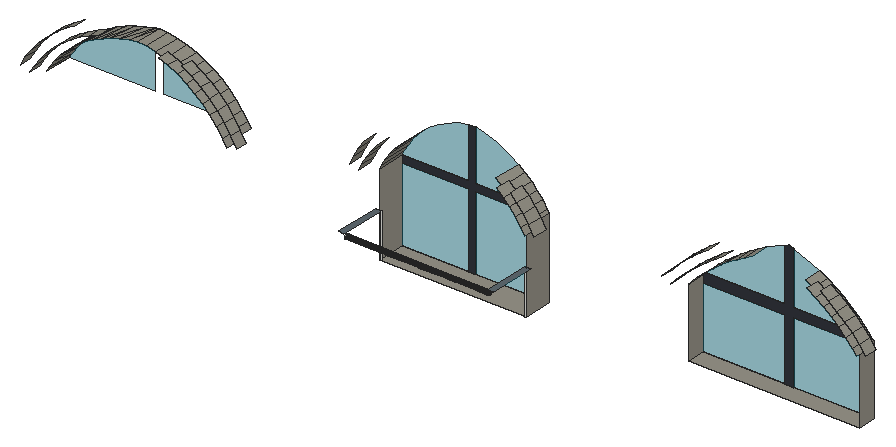
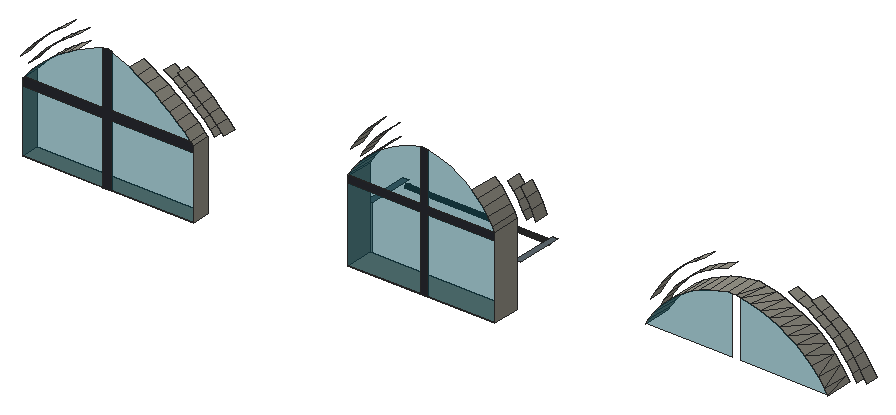
# SketchUp Ruby script. Lengths in inches.
U = 1.inch
M = Sketchup.active_model
def pt(a) = Geom::Point3d.new(a.map { |v| v * U })
def face(e, loops, mat)
  f = e.add_face(loops[0].map { |a| pt(a) })
  loops[1..].each { |l| e.add_face(l.map { |a| pt(a) }).erase! }
  f.material = f.back_material = mat if mat
  f
end
# faces: each face lists its corners as indices into pts; further lists are holes
def faces(e, pts, list, mat = nil) = list.each { |f| face(e, (f[0].is_a?(Array) ? f : [f]).map { |l| l.map { |i| pts[i] } }, mat) }
# xy, xz, yz: faces in a plane at the given z, y or x. An outline is a flat list of corners, or four numbers for a rectangle; further outlines are holes
def ring(l) = l.size == 4 ? [[l[0], l[1]], [l[2], l[1]], [l[2], l[3]], [l[0], l[3]]] : l.each_slice(2).to_a
def flat(e, list, mat, &to3) = list.each { |f| face(e, (f[0].is_a?(Array) ? f : [f]).map { |l| ring(l).map { |u, v| to3.(u, v) } }, mat) }
def xy(e, z, list, mat = nil) = flat(e, list, mat) { |x, y| [x, y, z] }
def xz(e, y, list, mat = nil) = flat(e, list, mat) { |x, z| [x, y, z] }
def yz(e, x, list, mat = nil) = flat(e, list, mat) { |y, z| [x, y, z] }
def lines(e, pts, list) = list.each { |a, b| e.add_line(pt(pts[a]), pt(pts[b])) }
# prism: a flat outline (further loops are holes) pulled along v
def prism(e, loops, v, mat = nil)
  f = face(e, loops, mat); d = Geom::Vector3d.new(v.map { |x| x * U })
  f.pushpull(f.normal.samedirection?(d) ? d.length : -d.length)
end
def box(e, o, s, mat = nil) = prism(e, [[o, [o[0] + s[0], o[1], o[2]], [o[0] + s[0], o[1] + s[1], o[2]], [o[0], o[1] + s[1], o[2]]]], [0, 0, s[2]], mat)
def at(x, y, z, deg = 0) = Geom::Transformation.translation(pt([x, y, z])) * Geom::Transformation.rotation(ORIGIN, Z_AXIS, deg.degrees)
def axes(o, x, y, z) = Geom::Transformation.new([*x, 0, *y, 0, *z, 0, *pt(o).to_a, 1])
def part(name) = M.definitions.add(name)
# library, detail: a bought-in or finely detailed component or shape, given as its bounding box
def library(name, o, s) = part(name).tap { |d| box(d.entities, o, s) }
def detail(e, o, s) = box(e.add_group.entities, o, s)
def put(e, d, t, mat = nil) = e.add_instance(d, t).tap { |i| i.material = mat if mat }
def group(e, t, mat = nil) = e.add_group.tap { |g| g.transformation = t; g.material = mat if mat }.entities
root = M.entities
M.materials.add("[Color M07]").color = [58, 58, 58]
M.materials.add("[Formica Graystone]").color = [149, 146, 135]
M.materials.add("[Formica Laminate Dark]").color = [50, 53, 60]
M.materials.add("[Formica Speckled Grey]").color = [94, 105, 111]
M.materials.add("[Translucent Glass Tinted]").color = [4, 106, 127]
M.materials["[Translucent Glass Tinted]"].alpha = 0.48
xy(root,336.52,[[366.31,158.3,451.49,167.05]],"[Formica Graystone]")
xy(root,337.93,[[223.375,144.04,296.73,158.1]],"[Formica Graystone]")
xy(root,357.6,[[226.04,121.51,226.22,121.51,226.4,121.55,226.55,121.64,226.68,121.76,226.77,121.92,226.82,122.09,226.82,122.27,226.78,122.45,226.6875,122.6,226.5625,122.73,226.41,122.82,226.23,122.87,226.06,122.87,225.88,122.83,225.73,122.74,225.6,122.61,225.51,122.46,225.46,122.28,225.46,122.11,225.5,121.93,225.59,121.78,225.71,121.65,225.87,121.56]])
xy(root,357.67,[[291.54,121.51,291.72,121.51,291.9,121.55,292.05,121.64,292.18,121.76,292.27,121.92,292.32,122.09,292.32,122.27,292.28,122.45,292.1875,122.6,292.0625,122.73,291.91,122.82,291.73,122.87,291.56,122.87,291.38,122.83,291.23,122.74,291.1,122.61,291.01,122.46,290.96,122.28,290.96,122.11,291,121.93,291.09,121.78,291.21,121.65,291.37,121.56]])
xy(root,357.79,[[248.54,121.51,248.72,121.51,248.9,121.55,249.05,121.64,249.18,121.76,249.27,121.92,249.32,122.09,249.32,122.27,249.28,122.45,249.1875,122.6,249.0625,122.73,248.91,122.82,248.73,122.87,248.56,122.87,248.38,122.83,248.23,122.74,248.1,122.61,248.01,122.46,247.96,122.28,247.96,122.11,248,121.93,248.09,121.78,248.21,121.65,248.37,121.56]])
xy(root,357.82,[[288.85,121.51,289.03,121.51,289.21,121.55,289.36,121.64,289.49,121.76,289.58,121.92,289.63,122.09,289.63,122.27,289.59,122.45,289.5,122.6,289.375,122.73,289.22,122.82,289.05,122.87,288.87,122.87,288.69,122.83,288.54,122.74,288.41,122.61,288.32,122.46,288.27,122.28,288.27,122.11,288.3125,121.93,288.4,121.78,288.53,121.65,288.68,121.56]])
xy(root,358.04,[[294.1,121.51,294.28,121.51,294.46,121.55,294.61,121.64,294.74,121.76,294.83,121.92,294.88,122.09,294.88,122.27,294.84,122.45,294.75,122.6,294.625,122.73,294.47,122.82,294.3,122.87,294.12,122.87,293.94,122.83,293.79,122.74,293.66,122.61,293.57,122.46,293.52,122.28,293.52,122.11,293.5625,121.93,293.65,121.78,293.78,121.65,293.93,121.56]])
xy(root,358.07,[[228.85,121.51,229.03,121.51,229.21,121.55,229.36,121.64,229.49,121.76,229.58,121.92,229.63,122.09,229.63,122.27,229.59,122.45,229.5,122.6,229.375,122.73,229.22,122.82,229.05,122.87,228.87,122.87,228.69,122.83,228.54,122.74,228.41,122.61,228.32,122.46,228.27,122.28,228.27,122.11,228.3125,121.93,228.4,121.78,228.53,121.65,228.68,121.56],[242.92,121.51,243.1,121.51,243.27,121.55,243.43,121.64,243.55,121.76,243.65,121.92,243.69,122.09,243.7,122.27,243.65,122.45,243.5625,122.6,243.4375,122.73,243.28,122.82,243.11,122.87,242.93,122.87,242.76,122.83,242.6,122.74,242.47,122.61,242.38,122.46,242.33,122.28,242.33,122.11,242.375,121.93,242.46,121.78,242.59,121.65,242.74,121.56],[245.73,121.51,245.91,121.51,246.08,121.55,246.24,121.64,246.37,121.76,246.46,121.92,246.51,122.09,246.51,122.27,246.46,122.45,246.375,122.6,246.25,122.73,246.1,122.82,245.92,122.87,245.74,122.87,245.57,122.83,245.41,122.74,245.28,122.61,245.19,122.46,245.15,122.28,245.14,122.11,245.1875,121.93,245.28,121.78,245.4,121.65,245.56,121.56],[251.29,121.51,251.47,121.51,251.65,121.55,251.8,121.64,251.93,121.76,252.02,121.92,252.07,122.09,252.07,122.27,252.03,122.45,251.9375,122.6,251.8125,122.73,251.66,122.82,251.48,122.87,251.31,122.87,251.13,122.83,250.98,122.74,250.85,122.61,250.76,122.46,250.71,122.28,250.71,122.11,250.75,121.93,250.84,121.78,250.96,121.65,251.12,121.56],[267.79,121.51,267.97,121.51,268.15,121.55,268.3,121.64,268.43,121.76,268.52,121.92,268.57,122.09,268.57,122.27,268.53,122.45,268.4375,122.6,268.3125,122.73,268.16,122.82,267.98,122.87,267.81,122.87,267.63,122.83,267.48,122.74,267.35,122.61,267.26,122.46,267.21,122.28,267.21,122.11,267.25,121.93,267.34,121.78,267.46,121.65,267.62,121.56],
  [270.54,121.51,270.72,121.51,270.9,121.55,271.05,121.64,271.18,121.76,271.27,121.92,271.32,122.09,271.32,122.27,271.28,122.45,271.1875,122.6,271.0625,122.73,270.91,122.82,270.73,122.87,270.56,122.87,270.38,122.83,270.23,122.74,270.1,122.61,270.01,122.46,269.96,122.28,269.96,122.11,270,121.93,270.09,121.78,270.21,121.65,270.37,121.56],[273.48,121.51,273.66,121.51,273.83,121.55,273.99,121.64,274.12,121.76,274.21,121.92,274.26,122.09,274.26,122.27,274.21,122.45,274.125,122.6,274,122.73,273.85,122.82,273.67,122.87,273.49,122.87,273.32,122.83,273.16,122.74,273.03,122.61,272.94,122.46,272.9,122.28,272.89,122.11,272.9375,121.93,273.03,121.78,273.15,121.65,273.31,121.56],[285.92,121.51,286.1,121.51,286.27,121.55,286.43,121.64,286.55,121.76,286.65,121.92,286.69,122.09,286.7,122.27,286.65,122.45,286.5625,122.6,286.4375,122.73,286.28,122.82,286.11,122.87,285.93,122.87,285.76,122.83,285.6,122.74,285.47,122.61,285.38,122.46,285.33,122.28,285.33,122.11,285.375,121.93,285.46,121.78,285.59,121.65,285.74,121.56]])
xy(root,358.23,[[279.04,121.51,279.22,121.51,279.4,121.55,279.55,121.64,279.68,121.76,279.77,121.92,279.82,122.09,279.82,122.27,279.78,122.45,279.6875,122.6,279.5625,122.73,279.41,122.82,279.23,122.87,279.06,122.87,278.88,122.83,278.73,122.74,278.6,122.61,278.51,122.46,278.46,122.28,278.46,122.11,278.5,121.93,278.59,121.78,278.71,121.65,278.87,121.56]])
xy(root,358.31,[[231.67,121.51,231.85,121.51,232.02,121.55,232.18,121.64,232.3,121.76,232.4,121.92,232.44,122.09,232.45,122.27,232.4,122.45,232.3125,122.6,232.1875,122.73,232.03,122.82,231.86,122.87,231.68,122.87,231.51,122.83,231.35,122.74,231.22,122.61,231.13,122.46,231.08,122.28,231.08,122.11,231.125,121.93,231.21,121.78,231.34,121.65,231.49,121.56],[234.48,121.51,234.66,121.51,234.83,121.55,234.99,121.64,235.12,121.76,235.21,121.92,235.26,122.09,235.26,122.27,235.21,122.45,235.125,122.6,235,122.73,234.85,122.82,234.67,122.87,234.49,122.87,234.32,122.83,234.16,122.74,234.03,122.61,233.94,122.46,233.9,122.28,233.89,122.11,233.9375,121.93,234.03,121.78,234.15,121.65,234.31,121.56],[254.04,121.51,254.22,121.51,254.4,121.55,254.55,121.64,254.68,121.76,254.77,121.92,254.82,122.09,254.82,122.27,254.78,122.45,254.6875,122.6,254.5625,122.73,254.41,122.82,254.23,122.87,254.06,122.87,253.88,122.83,253.73,122.74,253.6,122.61,253.51,122.46,253.46,122.28,253.46,122.11,253.5,121.93,253.59,121.78,253.71,121.65,253.87,121.56],[256.79,121.51,256.97,121.51,257.15,121.55,257.3,121.64,257.43,121.76,257.52,121.92,257.57,122.09,257.57,122.27,257.53,122.45,257.4375,122.6,257.3125,122.73,257.16,122.82,256.98,122.87,256.81,122.87,256.63,122.83,256.48,122.74,256.35,122.61,256.26,122.46,256.21,122.28,256.21,122.11,256.25,121.93,256.34,121.78,256.46,121.65,256.62,121.56],[259.54,121.51,259.72,121.51,259.9,121.55,260.05,121.64,260.18,121.76,260.27,121.92,260.32,122.09,260.32,122.27,260.28,122.45,260.1875,122.6,260.0625,122.73,259.91,122.82,259.73,122.87,259.56,122.87,259.38,122.83,259.23,122.74,259.1,122.61,259.01,122.46,258.96,122.28,258.96,122.11,259,121.93,259.09,121.78,259.21,121.65,259.37,121.56],
  [262.29,121.51,262.47,121.51,262.65,121.55,262.8,121.64,262.93,121.76,263.02,121.92,263.07,122.09,263.07,122.27,263.03,122.45,262.9375,122.6,262.8125,122.73,262.66,122.82,262.48,122.87,262.31,122.87,262.13,122.83,261.98,122.74,261.85,122.61,261.76,122.46,261.71,122.28,261.71,122.11,261.75,121.93,261.84,121.78,261.96,121.65,262.12,121.56],[282.29,121.51,282.47,121.51,282.65,121.55,282.8,121.64,282.93,121.76,283.02,121.92,283.07,122.09,283.07,122.27,283.03,122.45,282.9375,122.6,282.8125,122.73,282.66,122.82,282.48,122.87,282.31,122.87,282.13,122.83,281.98,122.74,281.85,122.61,281.76,122.46,281.71,122.28,281.71,122.11,281.75,121.93,281.84,121.78,281.96,121.65,282.12,121.56]])
xy(root,358.53,[[237.29,121.51,237.47,121.51,237.65,121.55,237.8,121.64,237.93,121.76,238.02,121.92,238.07,122.09,238.07,122.27,238.03,122.45,237.9375,122.6,237.8125,122.73,237.66,122.82,237.48,122.87,237.31,122.87,237.13,122.83,236.98,122.74,236.85,122.61,236.76,122.46,236.71,122.28,236.71,122.11,236.75,121.93,236.84,121.78,236.96,121.65,237.12,121.56],[240.1,121.51,240.28,121.51,240.46,121.55,240.61,121.64,240.74,121.76,240.83,121.92,240.88,122.09,240.88,122.27,240.84,122.45,240.75,122.6,240.625,122.73,240.47,122.82,240.3,122.87,240.12,122.87,239.94,122.83,239.79,122.74,239.66,122.61,239.57,122.46,239.52,122.28,239.52,122.11,239.5625,121.93,239.65,121.78,239.78,121.65,239.93,121.56],[265.04,121.51,265.22,121.51,265.4,121.55,265.55,121.64,265.68,121.76,265.77,121.92,265.82,122.09,265.82,122.27,265.78,122.45,265.6875,122.6,265.5625,122.73,265.41,122.82,265.23,122.87,265.06,122.87,264.88,122.83,264.73,122.74,264.6,122.61,264.51,122.46,264.46,122.28,264.46,122.11,264.5,121.93,264.59,121.78,264.71,121.65,264.87,121.56],[276.29,121.51,276.47,121.51,276.65,121.55,276.8,121.64,276.93,121.76,277.02,121.92,277.07,122.09,277.07,122.27,277.03,122.45,276.9375,122.6,276.8125,122.73,276.66,122.82,276.48,122.87,276.31,122.87,276.13,122.83,275.98,122.74,275.85,122.61,275.76,122.46,275.71,122.28,275.71,122.11,275.75,121.93,275.84,121.78,275.96,121.65,276.12,121.56]])
xy(root,359.98,[[221.4,120.91,224.22,144.04],[295.92,120.91,298.73,144.04]],"[Formica Speckled Grey]")
xz(root,144.04,[[223.375,337.93,224.22,359.98],[295.92,337.93,296.73,359.98]])
xz(root,157.6,[[57.22,363.79,100.86,363.79,100.86,392.22,95.875,391.25,90.98,389.9,86.22,388.15,81.61,386.02,77.1875,383.53,72.98,380.69,69.01,377.52,65.32,374.05,61.91,370.28,58.82,366.26],[104.96,363.79,148.1,363.79,148.1,363.97,146.62,366.62,143.875,370.65,140.79,374.42,137.39,377.91,133.69,381.08,129.73,383.92,125.53,386.4,121.14,388.5,116.57,390.21,111.875,391.51,107.08,392.39,104.96,392.59]],"[Translucent Glass Tinted]")
xz(root,158.1,[[256.49,337.93,260.1,337.93,260.1,374.93,296.73,374.93,296.73,377.84,296.41,378.37,260.1,378.37,260.1,403.77,259.55,403.88,256.49,403.57,256.49,378.37,223.375,378.37,223.375,374.93,256.49,374.93]],"[Formica Laminate Dark]")
xz(root,158.1,[[223.375,337.93,256.49,374.93],[260.1,337.93,296.73,374.93],[223.375,378.37,256.49,378.37,256.49,403.57,252.47,402.78,248.55,401.61,244.76,400.07,241.125,398.18,237.6875,395.96,234.47,393.42,231.52,390.6,228.84,387.5,226.46,384.17,224.41,380.625],[260.1,378.37,296.41,378.37,295.73,379.52,293.33,382.9375,290.6875,386.17,287.8,389.1875,284.7,391.99,281.4,394.54,277.91,396.84,274.27,398.875,270.47,400.625,266.5625,402.09,262.55,403.25,260.1,403.77]],"[Translucent Glass Tinted]")
xz(root,167.05,[[407.09,336.52,411.36,336.52,411.36,367.77,451.49,367.77,451.49,371.35,450.74,372.28,411.36,372.28,411.36,398.78,409.2,399.41,407.09,398.63,407.09,372.28,367.48,372.28,366.31,371.02,366.31,367.77,407.09,367.77]],"[Formica Laminate Dark]")
xz(root,167.05,[[366.31,336.52,407.09,367.77],[411.36,336.52,451.49,367.77],[367.48,372.28,407.09,372.28,407.09,398.63,402.67,396.78,398.33,394.75,394.08,392.53,389.92,390.13,385.88,387.56,381.94,384.83,378.13,381.92,374.44,378.86,370.89,375.64],[411.36,372.28,450.74,372.28,450.21,372.9375,447.04,376.44,443.68,379.77,440.15,382.91,436.44,385.84,432.58,388.57,428.58,391.07,424.4375,393.36,420.18,395.41,415.8125,397.22,411.36,398.78]],"[Translucent Glass Tinted]")
yz(root,223.375,[[144.04,337.93,158.1,378.37]],"[Formica Graystone]")
yz(root,224.22,[[122.22,357.13,121.97,357.16,121.75,357.25,121.55,357.4,121.41,357.6,121.3125,357.82,121.28,358.07,121.3125,358.31,121.41,358.53,121.55,358.73,121.75,358.88,121.97,358.97,122.22,359,122.46,358.97,122.6875,358.88,122.88,358.73,123.03,358.53,123.125,358.31,123.16,358.07,123.125,357.82,123.03,357.6,122.88,357.4,122.6875,357.25,122.46,357.16]])
yz(root,296.73,[[144.04,337.93,158.1,377.84]],"[Formica Graystone]")
yz(root,366.31,[[158.3,336.52,167.05,371.02]],"[Formica Graystone]")
yz(root,451.49,[[158.3,336.52,167.05,371.35]],"[Formica Graystone]")
p = [[224.22,121.97,357.16],[224.22,122.22,357.13],[295.92,122.22,357.13],[295.92,121.97,357.16],[224.22,122.46,357.16],[295.92,122.46,357.16],
  [224.22,121.75,357.25],[295.92,121.75,357.25],[224.22,122.6875,357.25],[295.92,122.6875,357.25],[224.22,121.55,357.4],[295.92,121.55,357.4],
  [293.93,121.56,357.4],[291.37,121.56,357.4],[288.68,121.56,357.4],[285.74,121.56,357.4],[282.12,121.56,357.4],[278.87,121.56,357.4],
  [276.12,121.56,357.4],[273.31,121.56,357.4],[270.37,121.56,357.4],[267.62,121.56,357.4],[264.87,121.56,357.4],[262.12,121.56,357.4],
  [259.37,121.56,357.4],[256.62,121.56,357.4],[253.87,121.56,357.4],[251.12,121.56,357.4],[248.37,121.56,357.4],[245.56,121.56,357.4],
  [242.74,121.56,357.4],[239.93,121.56,357.4],[237.12,121.56,357.4],[234.31,121.56,357.4],[231.49,121.56,357.4],[228.68,121.56,357.4],
  [225.87,121.56,357.4],[224.22,122.88,357.4],[295.92,122.88,357.4],[224.22,121.41,357.6],[295.92,121.41,357.6],[224.22,123.03,357.6],
  [295.92,123.03,357.6],[224.22,121.3125,357.82],[295.92,121.3125,357.82],[224.22,123.125,357.82],[295.92,123.125,357.82],[224.22,121.28,358.07],
  [295.92,121.28,358.07],[224.22,123.16,358.07],[295.92,123.16,358.07],[224.22,121.3125,358.31],[295.92,121.3125,358.31],[224.22,123.125,358.31],
  [295.92,123.125,358.31],[224.22,121.41,358.53],[295.92,121.41,358.53],[224.22,123.03,358.53],[295.92,123.03,358.53],[224.22,121.55,358.73],
  [295.92,121.55,358.73],[224.22,122.88,358.73],[295.92,122.88,358.73],[224.22,121.75,358.88],[295.92,121.75,358.88],[224.22,122.6875,358.88],
  [295.92,122.6875,358.88],[224.22,121.97,358.97],[295.92,121.97,358.97],[224.22,122.46,358.97],[295.92,122.46,358.97],[224.22,122.22,359],
  [295.92,122.22,359],[57.22,144.04,363.79],[57.22,157.6,363.79],[58.7,144.04,366.21],[58.82,157.6,366.26],[148.1,144.04,363.97],
  [146.62,144.04,366.62],[146.62,157.6,366.62],[148.1,157.6,363.97],[53.67,144.04,364.79],[55.75,144.04,368.18],[55.75,138.29,368.18],
  [53.67,138.29,364.79],[149.64,144.04,368.49],[151.64,144.04,364.9],[151.64,138.29,364.9],[149.64,138.29,368.49],[51.64,144.04,370.94],
  [48.72,144.04,366.1875],[48.72,138.29,366.1875],[51.64,138.29,370.94],[156.59,144.04,366.1875],[153.85,144.04,371.09],[153.85,138.29,371.09],
  [156.59,138.29,366.1875],[61.59,144.04,370.16],[61.91,157.6,370.28],[143.875,144.04,370.65],[143.875,157.6,370.65],[58.81,144.04,372.37],
  [58.81,138.29,372.37],[146.72,144.04,372.77],[146.72,138.29,372.77],[64.78,144.04,373.87],[65.32,157.6,374.05],[140.79,144.04,374.42],
  [140.79,157.6,374.42],[54.92,144.04,375.45],[54.92,138.29,375.45],[367.48,158.3,372.28],[366.31,158.3,371.02],[366.31,167.05,371.02],
  [367.48,167.05,372.28],[150.69,144.04,375.74],[150.69,138.29,375.74],[451.49,158.3,371.35],[450.21,158.3,372.9375],[450.21,167.05,372.9375],
  [450.74,167.05,372.28],[451.49,167.05,371.35],[370.89,158.3,375.64],[370.89,167.05,375.64],[62.1875,144.04,376.29],[62.1875,138.29,376.29],
  [362.5,158.3,372.52],[364.75,158.3,374.93],[364.75,151.8,374.93],[362.5,151.8,372.52],[453.1,158.3,375.41],[455.3,158.3,372.69],
  [455.3,151.8,372.69],[453.1,151.8,375.41],[143.4375,144.04,376.79],[143.4375,138.29,376.79],[447.04,158.3,376.44],[447.04,167.05,376.44],
  [69.01,157.6,377.52],[68.26,144.04,377.31],[361.56,158.3,378.03],[358.05,158.3,374.26],[358.05,151.8,374.26],[361.56,151.8,378.03],
  [459.74,158.3,374.26],[456.48,158.3,378.3],[456.48,151.8,378.3],[459.74,151.8,374.26],[137.39,144.04,377.91],[137.39,157.6,377.91],
  [368.27,158.3,378.41],[368.27,151.8,378.41],[58.57,144.04,379.67],[58.57,138.29,379.67],[449.8,158.3,379.07],[449.8,151.8,379.07],
  [374.44,158.3,378.86],[374.44,167.05,378.86],[147.13,144.04,380.09],[147.13,138.29,380.09],[65.875,144.04,379.93],[65.875,138.29,379.93],
  [443.68,158.3,379.77],[443.68,167.05,379.77],[139.82,144.04,380.5],[139.82,138.29,380.5],[72.98,157.6,380.69],[72.01,144.04,380.45],
  [296.73,144.04,377.84],[295.73,144.04,379.52],[295.73,158.1,379.52],[296.41,158.1,378.37],[296.73,158.1,377.84],[133.69,144.04,381.08],
  [133.69,157.6,381.08],[365.22,158.3,381.64],[365.22,151.8,381.64],[453.01,158.3,382.14],[453.01,151.8,382.14],[224.41,144.04,380.625],
  [223.375,144.04,378.37],[223.375,158.1,378.37],[224.41,158.1,380.625],[371.95,158.3,381.74],[371.95,151.8,381.74],[378.13,158.3,381.92],
  [378.13,167.05,381.92],[299.68,144.04,382.07],[301.43,144.04,379.13],[301.43,136.91,379.13],[299.68,136.91,382.07],[446.29,158.3,382.55],
  [446.29,151.8,382.55],[218.68,144.04,379.39],[220.23,144.04,382.79],[220.23,136.91,382.79],[218.68,136.91,379.39],[293.33,144.04,382.9375],
  [293.33,158.1,382.9375],[62.54,144.04,383.59],[62.54,138.29,383.59],[440.15,158.3,382.91],[440.15,167.05,382.91],[69.84,144.04,383.26],
  [69.84,138.29,383.26],[143.21,144.04,384.11],[143.21,138.29,384.11],[216.07,144.04,384.94],[213.99,144.04,380.42],[213.99,136.91,380.42],
  [216.07,136.91,384.94],[306.11,144.04,380.42],[303.62,144.04,384.61],[303.62,136.91,384.61],[306.11,136.91,380.42],[135.88,144.04,383.875],
  [135.88,138.29,383.875],[77.1875,157.6,383.53],[76,144.04,383.29],[226.46,144.04,384.17],[226.46,158.1,384.17],[129.73,144.04,383.92],
  [129.73,157.6,383.92],[369.03,158.3,385.09],[369.03,151.8,385.09],[375.76,158.3,384.9],[375.76,151.8,384.9],[381.94,158.3,384.83],
  [381.94,167.05,384.83],[297.08,144.04,385.78],[297.08,136.91,385.78],[449.33,158.3,385.79],[449.33,151.8,385.79],[442.6,158.3,385.83],
  [442.6,151.8,385.83],[222.51,144.04,386.72],[222.51,136.91,386.72],[290.6875,144.04,386.17],[290.6875,158.1,386.17],[436.44,158.3,385.84],
  [436.44,167.05,385.84],[74.0625,144.04,386.26],[74.0625,138.29,386.26],[81.61,157.6,386.02],[80.2,144.04,385.79],[66.81,144.04,387.18],
  [66.81,138.29,387.18],[131.67,144.04,386.89],[131.67,138.29,386.89],[125.53,144.04,386.4],[125.53,157.6,386.4],[138.94,144.04,387.77],
  [138.94,138.29,387.77],[228.84,144.04,387.5],[228.84,158.1,387.5],[300.82,144.04,388.61],[300.82,136.91,388.61],[385.88,158.3,387.56],
  [385.88,167.05,387.56],[218.56,144.04,389.25],[218.56,136.91,389.25],[379.7,158.3,387.91],[379.7,151.8,387.91],[372.99,158.3,388.38],
  [372.99,151.8,388.38],[294.21,144.04,389.28],[294.21,136.91,389.28],[86.22,157.6,388.15],[84.59,144.04,387.95],[438.73,158.3,388.89],
  [438.73,151.8,388.89],[445.45,158.3,389.23],[445.45,151.8,389.23],[432.58,158.3,388.57],[432.58,167.05,388.57],[287.8,144.04,389.1875],
  [287.8,158.1,389.1875],[78.51,144.04,388.91],[78.51,138.29,388.91],[121.14,144.04,388.5],[121.14,157.6,388.5],[225.14,144.04,390.41],
  [225.14,136.91,390.41],[127.2,144.04,389.53],[127.2,138.29,389.53],[71.35,144.04,390.41],[71.35,138.29,390.41],[231.52,144.04,390.6],
  [231.52,158.1,390.6],[389.92,158.3,390.13],[389.92,167.05,390.13],[134.375,144.04,391.05],[134.375,138.29,391.05],[90.98,157.6,389.9],
  [89.14,144.04,389.75],[383.77,158.3,390.74],[383.77,151.8,390.74],[377.08,158.3,391.5],[377.08,151.8,391.5],[116.57,144.04,390.21],
  [116.57,157.6,390.21],[297.72,144.04,392.39],[297.72,136.91,392.39],[428.58,158.3,391.07],[428.58,167.05,391.07],[83.16,144.04,391.19],
  [83.16,138.29,391.19],[434.69,158.3,391.74],[434.69,151.8,391.74],[284.7,144.04,391.99],[284.7,158.1,391.99],[441.39,158.3,392.45],
  [441.39,151.8,392.45],[221.45,144.04,393.3125],[221.45,136.91,393.3125],[291.08,144.04,392.56],[291.08,136.91,392.56],[122.52,144.04,391.77],
  [122.52,138.29,391.77],[95.875,157.6,391.25],[93.83,144.04,391.17],[394.08,158.3,392.53],[394.08,167.05,392.53],[111.875,144.04,391.51],
  [111.875,157.6,391.51],[228.11,144.04,393.84],[228.11,136.91,393.84],[76.15,144.04,393.27],[76.15,138.29,393.27],[234.47,144.04,393.42],
  [234.47,158.1,393.42],[387.95,158.3,393.39],[387.95,151.8,393.39],[129.53,144.04,393.91],[129.53,138.29,393.91],[424.4375,158.3,393.36],
  [424.4375,167.05,393.36],[87.98,144.04,393.1],[87.98,138.29,393.1],[100.86,157.6,392.22],[98.61,144.04,392.22],[107.08,144.04,392.39],
  [107.08,157.6,392.39],[381.31,158.3,394.4375],[381.31,151.8,394.4375],[430.51,158.3,394.36],[430.51,151.8,394.36],[117.67,144.04,393.58],
  [117.67,138.29,393.58],[281.4,144.04,394.54],[281.4,158.1,394.54],[102.83,157.6,392.79],[102.83,144.04,392.79],[294.35,144.04,395.92],
  [294.35,136.91,395.92],[104.96,157.6,392.59],[437.15,158.3,395.44],[437.15,151.8,395.44],[398.33,158.3,394.75],[398.33,167.05,394.75],
  [287.72,144.04,395.59],[287.72,136.91,395.59]]
faces(root,p,[[0,1,2,3],[1,4,5,2],[6,0,3,7],[4,8,9,5],[10,6,7,11,12,13,14,15,16,17,18,19,20,21,22,23,24,25,26,27,28,29,30,31,32,33,34,35,36],[8,37,38,9],[39,10,36,35,34,33,32,31,30,29,28,27,26,25,24,23,22,21,20,19,18,17,16,15,14,13,12,11,40],[37,41,42,38],
  [43,39,40,44],[41,45,46,42],[47,43,44,48],[45,49,50,46],[51,47,48,52],[49,53,54,50],[55,51,52,56],[53,57,58,54],
  [59,55,56,60],[57,61,62,58],[63,59,60,64],[61,65,66,62],[67,63,64,68],[65,69,70,66],[71,67,68,72],[69,71,72,70]],"[Color M07]")
faces(root,p,[[73,74,75],[76,75,74],[77,78,79,80],[81,82,83,84],[85,86,87,88],[89,90,91,92],[93,94,95,96],[75,76,97],
  [98,97,76],[78,99,100,79],[82,101,102,83],[103,85,88,104],[97,98,105],[106,105,98],[99,107,108,100],[109,89,92,110],
  [111,112,113,114],[94,115,116,95],[117,118,119,120,121],[122,111,114,123],[101,124,125,102],[126,127,128,129],[130,131,132,133],[134,103,104,135],
  [118,136,137,119],[106,138,105],[139,105,138],[140,141,142,143],[144,145,146,147],[107,148,149,108],[127,150,151,128],[152,109,110,153],
  [154,130,133,155],[156,122,123,157],[115,158,159,116],[124,160,161,125],[136,162,163,137],[164,134,135,165],[138,166,139],[167,139,166],
  [168,169,170,171,172],[148,173,174,149],[175,140,143,176],[145,177,178,146],[179,180,181,182],[150,183,184,151],[185,156,157,186],[187,188,189,190],
  [191,154,155,192],[193,194,195,196],[169,197,198,170],[199,152,153,200],[162,201,202,163],[160,203,204,161],[158,205,206,159],[207,208,209,210],
  [211,212,213,214],[215,164,165,216],[166,217,167],[218,167,217],[219,179,182,220],[173,221,222,174],[223,175,176,224],[183,225,226,184],
  [227,185,186,228],[229,187,190,230],[177,231,232,178],[233,191,192,234],[194,235,236,195],[197,237,238,198],[201,239,240,202],[203,241,242,204],
  [217,243,218],[244,218,243],[245,199,200,246],[247,215,216,248],[221,249,250,222],[205,251,252,206],[253,219,220,254],[212,255,256,213],
  [257,227,228,258],[259,207,210,260],[225,261,262,226],[263,223,224,264],[265,229,230,266],[243,267,244],[268,244,267],[269,233,234,270],
  [231,271,272,232],[239,273,274,240],[237,275,276,238],[241,277,278,242],[249,279,280,250],[235,281,282,236],[283,247,248,284],[285,245,246,286],
  [287,253,254,288],[289,257,258,290],[251,291,292,252],[267,293,268],[294,268,293],[261,295,296,262],[297,263,264,298],[279,299,300,280],
  [255,301,302,256],[273,303,304,274],[277,305,306,278],[307,269,270,308],[275,309,310,276],[271,311,312,272],[313,259,260,314],[315,265,266,316],
  [317,283,284,318],[293,319,294],[320,294,319],[321,289,290,322],[299,323,324,300],[281,325,326,282],[327,285,286,328],[329,287,288,330],
  [295,331,332,296],[291,333,334,292],[303,335,336,304],[305,337,338,306],[319,339,320],[340,320,339],[323,341,342,324],[343,297,298,344],
  [345,307,308,346],[347,317,318,348],[309,349,350,310],[339,351,340],[352,340,351],[301,353,354,302],[351,355,342,341,352],[311,356,357,312],
  [358,321,322,359],[360,315,316,361]],"[Formica Graystone]")
